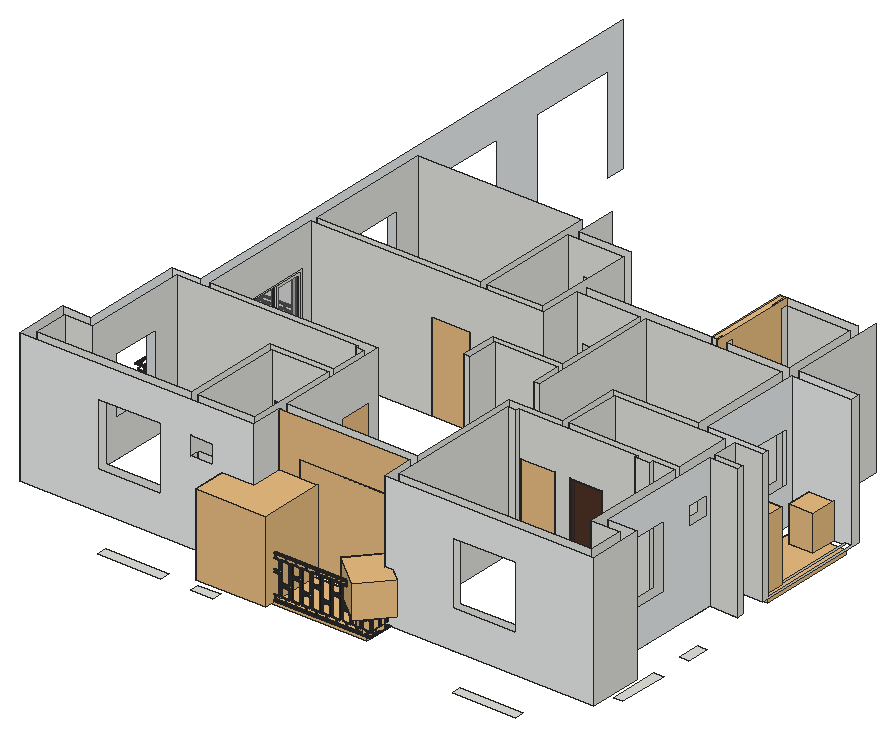
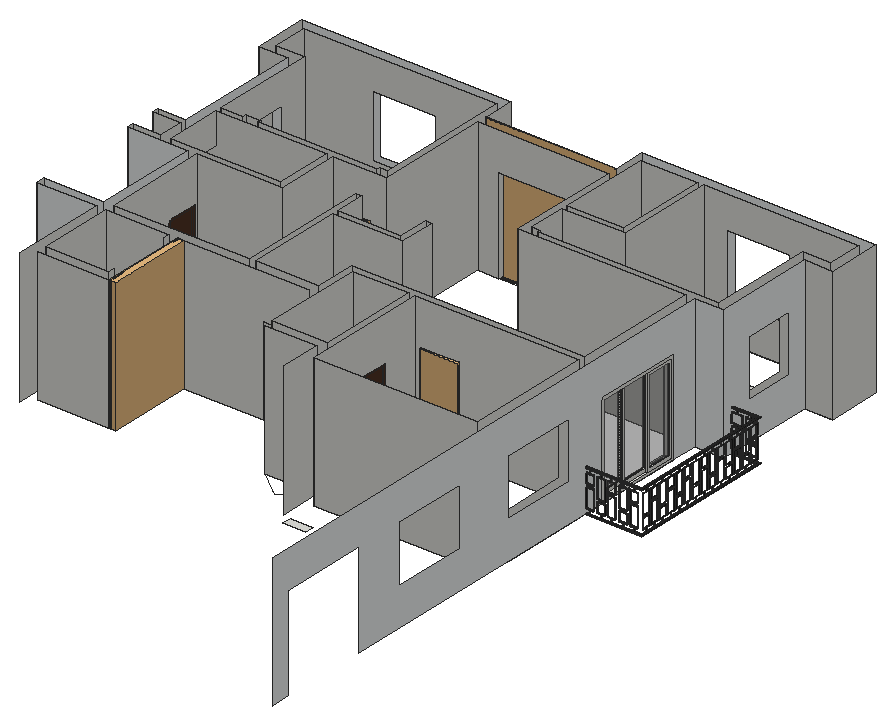
# SketchUp Ruby script. Lengths in inches.
U = 1.inch
M = Sketchup.active_model
def pt(a) = Geom::Point3d.new(a.map { |v| v * U })
def face(e, loops, mat)
  f = e.add_face(loops[0].map { |a| pt(a) })
  loops[1..].each { |l| e.add_face(l.map { |a| pt(a) }).erase! }
  f.material = f.back_material = mat if mat
  f
end
# faces: each face lists its corners as indices into pts; further lists are holes
def faces(e, pts, list, mat = nil) = list.each { |f| face(e, (f[0].is_a?(Array) ? f : [f]).map { |l| l.map { |i| pts[i] } }, mat) }
# xy, xz, yz: faces in a plane at the given z, y or x. An outline is a flat list of corners, or four numbers for a rectangle; further outlines are holes
def ring(l) = l.size == 4 ? [[l[0], l[1]], [l[2], l[1]], [l[2], l[3]], [l[0], l[3]]] : l.each_slice(2).to_a
def flat(e, list, mat, &to3) = list.each { |f| face(e, (f[0].is_a?(Array) ? f : [f]).map { |l| ring(l).map { |u, v| to3.(u, v) } }, mat) }
def xy(e, z, list, mat = nil) = flat(e, list, mat) { |x, y| [x, y, z] }
def xz(e, y, list, mat = nil) = flat(e, list, mat) { |x, z| [x, y, z] }
def yz(e, x, list, mat = nil) = flat(e, list, mat) { |y, z| [x, y, z] }
def lines(e, pts, list) = list.each { |a, b| e.add_line(pt(pts[a]), pt(pts[b])) }
# prism: a flat outline (further loops are holes) pulled along v
def prism(e, loops, v, mat = nil)
  f = face(e, loops, mat); d = Geom::Vector3d.new(v.map { |x| x * U })
  f.pushpull(f.normal.samedirection?(d) ? d.length : -d.length)
end
def box(e, o, s, mat = nil) = prism(e, [[o, [o[0] + s[0], o[1], o[2]], [o[0] + s[0], o[1] + s[1], o[2]], [o[0], o[1] + s[1], o[2]]]], [0, 0, s[2]], mat)
def at(x, y, z, deg = 0) = Geom::Transformation.translation(pt([x, y, z])) * Geom::Transformation.rotation(ORIGIN, Z_AXIS, deg.degrees)
def axes(o, x, y, z) = Geom::Transformation.new([*x, 0, *y, 0, *z, 0, *pt(o).to_a, 1])
def part(name) = M.definitions.add(name)
# library, detail: a bought-in or finely detailed component or shape, given as its bounding box
def library(name, o, s) = part(name).tap { |d| box(d.entities, o, s) }
def detail(e, o, s) = box(e.add_group.entities, o, s)
def put(e, d, t, mat = nil) = e.add_instance(d, t).tap { |i| i.material = mat if mat }
def group(e, t, mat = nil) = e.add_group.tap { |g| g.transformation = t; g.material = mat if mat }.entities
root = M.entities
M.materials.add("02 - Default").color = [196, 209, 187]
M.materials.add("02 - DefaultW").color = [91, 118, 29]
M.materials.add("04 - Default").color = [38, 38, 38]
M.materials.add("04 - DefaultW").color = [92, 55, 26]
M.materials.add("06 - Default").color = [255, 255, 255]
M.materials.add("07 - Default").color = [92, 55, 26]
M.materials.add("10 - Default").color = [62, 56, 39]
M.materials.add("Polis06_194").color = [79, 50, 36]
M.materials.add("[3P0081_White-City]").color = [235, 238, 238]
M.materials.add("[Color M00]").color = [255, 255, 255]
M.materials.add("[Color M08]").color = [30, 30, 30]
M.materials.add("[Translucent Glass Gray]").color = [128, 128, 128]
M.materials["[Translucent Glass Gray]"].alpha = 0.5
c1 = part("Group\#70")
prism(c1.entities,[[[4.13,0,3.9375],[7.875,0,3.9375],[7.875,0,13.78],[4.13,0,13.78],[4.13,0,15.75],[7.875,0,15.75],[7.875,0,35.43],[4.13,0,35.43],[4.13,0,39.37],[3.74,0,39.37],[3.74,0,35.43],[0,0,35.43],[0,0,15.75],[3.74,0,15.75],[3.74,0,13.78],[0,0,13.78],[0,0,3.9375],[3.74,0,3.9375],[3.74,0,0],[4.13,0,0]],[[0.39,0,16.14],[0.39,0,35.04],[7.48,0,35.04],[7.48,0,16.14]],[[7.48,0,4.33],[0.39,0,4.33],[0.39,0,13.39],[7.48,0,13.39]]],[0,0.39,0],"[Color M08]")
c2 = part("Group\#69")
prism(c2.entities,[[[3.74,0,35.43],[0,0,35.43],[0,0,25.59],[3.74,0,25.59],[3.74,0,23.62],[0,0,23.62],[0,0,3.9375],[3.74,0,3.9375],[3.74,0,0],[4.13,0,0],[4.13,0,3.9375],[7.875,0,3.9375],[7.875,0,23.62],[4.13,0,23.62],[4.13,0,25.59],[7.875,0,25.59],[7.875,0,35.43],[4.13,0,35.43],[4.13,0,39.37],[3.74,0,39.37]],[[7.48,0,23.23],[7.48,0,4.33],[0.39,0,4.33],[0.39,0,23.23]],[[0.39,0,35.04],[7.48,0,35.04],[7.48,0,25.98],[0.39,0,25.98]]],[0,0.39,0],"[Color M08]")
c3 = part("Group\#71")
put(c3.entities,c1,at(0,0,0))
put(c3.entities,c2,at(9.84,0,0))
c4 = part("Group\#81")
g1 = group(c4.entities,at(0,0,0))
prism(g1,[[[24,-19.7,0],[0,-19.7,0],[0,120.08,0],[24,120.08,0],[24,118.11,0],[1.97,118.11,0],[1.97,-17.76,0],[24,-17.76,0]]],[0,0,0.79],"[Color M08]")
put(c4.entities,c3,axes([0.79,40.35,0.79],[0,1,0],[1,0,0],[0,0,1]))
put(c4.entities,c3,at(2.95,118.9,0.79))
put(c4.entities,c3,axes([0.79,79.72,0.79],[0,1,0],[1,0,0],[0,0,1]))
put(c4.entities,c3,axes([0.79,60.04,0.79],[0,1,0],[1,0,0],[0,0,1]))
put(c4.entities,c3,axes([0.79,99.41,0.79],[0,1,0],[1,0,0],[0,0,1]))
put(c4.entities,c3,axes([0.79,0.98,0.79],[0,1,0],[1,0,0],[0,0,1]))
g2 = group(c4.entities,at(0,0,40.16))
prism(g2,[[[24,-19.7,0],[0,-19.7,0],[0,120.08,0],[24,120.08,0],[24,118.11,0],[1.97,118.11,0],[1.97,-17.76,0],[24,-17.76,0]]],[0,0,0.79],"[Color M08]")
put(c4.entities,c3,axes([0.79,20.67,0.79],[0,1,0],[1,0,0],[0,0,1]))
put(c4.entities,c3,axes([0.79,-18.7,0.79],[0,1,0],[1,0,0],[0,0,1]))
put(c4.entities,c3,axes([2.95,-18.49,0.79],[1,0,0],[0,-1,0],[0,0,1]))
c5 = library("MONSTERA_Defintion",[-100.72,-132.16,0],[226.75,232.88,1000])
c6 = library("MONSTERA_Defintion1",[-382.23,-503.1,29.34],[811.96,1000,773.77])
c7 = library("POT_Defintion",[-467.71,-467.71,0],[935.42,935.42,1000])
c8 = library("POT_Defintion6",[-504.36,-499.05,1069.94],[1000,1000,51.81])
c9 = library("TABLE_Defintion5",[-349.98,-500,-99.29],[912.18,1000,162.92])
c10 = library("TABLE_Defintion3",[-282.7,-491.23,-690.5],[848.82,1000,669.35])
c11 = library("TABLE_Defintion",[-354.24,-500,-9.27],[914.7,1000,77.28])
c12 = part("Monstera Plant 50")
g3 = group(c12.entities,at(0,0,0))
g4 = group(g3,at(0,0,0))
put(g4,c5,axes([-70.21,316.62,1332.52],[0.60525,0.72131,0],[-0.72131,0.60525,0],[0,0,0.92363]),"02 - DefaultW")
put(g4,c6,axes([-70.21,316.62,1332.52],[2.09136,2.49238,0],[-2.49238,2.09136,0],[0,0,3.1915]),"02 - Default")
g5 = group(c12.entities,at(0,0,0))
g6 = group(g5,at(0,0,0))
put(g6,c7,axes([-63.73,311.08,962.21],[0.47902,0.57088,0],[-0.57088,0.47902,0],[0,0,0.69328]),"04 - Default")
put(g6,c8,axes([-63.73,311.08,962.21],[0.41695,0.4969,0],[-0.4969,0.41695,0],[0,0,0.60345]),"10 - Default")
g7 = group(c12.entities,at(0,0,0))
g8 = group(g7,at(0,0,0))
put(g8,c9,axes([-8.95,303.3125,886.6],[1.07163,-0.6187,0],[0.6187,1.07163,0],[0,0,1.23741]),"04 - DefaultW")
put(g8,c10,axes([-8.95,303.3125,886.6],[1.11435,-0.64337,0],[0.64337,1.11435,0],[0,0,1.28674]),"07 - Default")
put(g8,c11,axes([-8.95,303.3125,886.6],[1.10303,-0.63684,0],[0.63684,1.10303,0],[0,0,1.27367]),"06 - Default")
c13 = library("Flora+17",[-57.52,158.6,-38.64],[66.99,62.88,77.28])
c14 = library("Floor panel",[0,13.98,-0.38],[148.62,177.51,16.92])
c15 = library("Group\#241",[0,-0.25,0],[124.5,0.25,126])
c16 = library("SLIDING+GLASS+DOOR",[0,-0.75,0],[72,5.75,80])
c17 = part("Flush door")
xy(c17.entities,0,[[0,0,4.72,1.18],[0,34.25,4.72,35.43]],"Polis06_194")
xy(c17.entities,85.26,[[0,1.18,4.72,34.25]],"Polis06_194")
xy(c17.entities,86.61,[[0,0,4.72,35.43]],"Polis06_194")
xz(c17.entities,0,[[0,0,4.72,86.61]],"Polis06_194")
xz(c17.entities,1.18,[[0,0,2.36,85.26],[2.36,0,4.72,85.26]],"Polis06_194")
xz(c17.entities,34.25,[[0,0,4.72,85.26]],"Polis06_194")
xz(c17.entities,35.43,[[0,0,4.72,86.61]],"Polis06_194")
yz(c17.entities,0,[[0,0,1.18,86.61],[34.25,0,35.43,86.61],[1.18,85.26,34.25,86.61]],"Polis06_194")
yz(c17.entities,2.36,[[1.18,0,34.25,0,34.25,85.21,1.18,85.26]],"Polis06_194")
yz(c17.entities,4.72,[[0,0,1.18,86.61],[34.25,0,35.43,86.61],[1.18,85.26,34.25,86.61]],"Polis06_194")
c18 = library("PINTU 6 YA",[0,-0.6875,0],[35.83,8.07,80.71])
c19 = part("Group\#75")
put(c19.entities,c1,at(0,0,0))
put(c19.entities,c2,at(9.84,0,0))
c20 = part("Group\#76")
put(c20.entities,c1,at(0,0,0))
put(c20.entities,c2,at(9.84,0,0))
c21 = part("Group\#74")
put(c21.entities,c19,axes([0.79,60.04,0.79],[0,1,0],[1,0,0],[0,0,1]))
put(c21.entities,c19,axes([0.79,40.35,0.79],[0,1,0],[1,0,0],[0,0,1]))
put(c21.entities,c19,axes([0.79,79.72,0.79],[0,1,0],[1,0,0],[0,0,1]))
g9 = group(c21.entities,at(0,0,40.16))
prism(g9,[[[54,-20.92,0],[0,-20.92,0],[0,120.08,0],[27,120.08,0],[27,118.11,0],[1.97,118.11,0],[1.97,-18.98,0],[54,-18.98,0]]],[0,0,0.79],"[Color M08]")
put(c21.entities,c20,axes([0.79,0.98,0.79],[0,1,0],[1,0,0],[0,0,1]))
put(c21.entities,c19,axes([0.79,20.67,0.79],[0,1,0],[1,0,0],[0,0,1]))
put(c21.entities,c19,axes([2.95,118.9,0.79],[1.35733,0,0],[0,1,0],[0,0,1]))
g10 = group(c21.entities,at(0,0,0))
prism(g10,[[[54,-20.92,0],[0,-20.92,0],[0,120.08,0],[27,120.08,0],[27,118.11,0],[1.97,118.11,0],[1.97,-18.98,0],[54,-18.98,0]]],[0,0,0.79],"[Color M08]")
put(c21.entities,c3,axes([0.79,99.41,0.79],[0,1,0],[1,0,0],[0,0,1]))
put(c21.entities,c20,axes([0.79,-18.7,0.79],[0,1,0],[1,0,0],[0,0,1]))
put(c21.entities,c20,axes([22.01,-20.17,0.79],[-1,0,0],[0,1,0],[0,0,1]))
g11 = group(c21.entities,at(43.22,-20.17,0.79))
put(g11,c1,axes([0,0,0],[-1,0,0],[0,1,0],[0,0,1]))
put(g11,c2,axes([-9.84,0,0],[-1,0,0],[0,1,0],[0,0,1]))
put(g11,c2,axes([10.78,0,0],[-1,0,0],[0,1,0],[0,0,1]))
c22 = part("구성 요소\#2")
prism(c22.entities,[[[0,0,0],[118.11,0,0],[118.11,0,78.74],[0,0,78.74]],[[116.14,0,76.77],[116.14,0,1.97],[1.97,0,1.97],[1.97,0,76.77]]],[0,7.875,0])
c23 = part("구성 요소\#1")
xy(c23.entities,0,[[[0,0,40.16,74.8],[2.375,2.375,37.78,72.43]]])
xy(c23.entities,1.18,[[2.375,2.375,37.78,72.43]],"[Translucent Glass Gray]")
xy(c23.entities,2.36,[[[0,0,40.16,74.8],[2.375,2.375,37.78,72.43]]])
xz(c23.entities,0,[[0,0,40.16,2.36]],"[Color M00]")
xz(c23.entities,2.375,[[2.375,0,37.78,1.18],[2.375,1.18,37.78,2.36]])
xz(c23.entities,72.43,[[2.375,0,37.78,1.18],[2.375,1.18,37.78,2.36]])
xz(c23.entities,74.8,[[0,0,40.16,2.36]],"[Color M00]")
yz(c23.entities,0,[[0,0,74.8,2.36]])
yz(c23.entities,2.375,[[2.375,0,72.43,1.18],[2.375,1.18,72.43,2.36]])
yz(c23.entities,37.78,[[2.375,0,72.43,1.18],[2.375,1.18,72.43,2.36]])
yz(c23.entities,40.16,[[0,0,74.8,2.36]])
c24 = part("구성 요소\#3")
xy(c24.entities,0,[[0,0,40.16,2.36]],"[Color M00]")
xy(c24.entities,2.375,[[2.375,0,37.78,1.18],[2.375,1.18,37.78,2.36]])
xy(c24.entities,35.83,[[38.48,0,39.47,0.39]])
xy(c24.entities,35.83,[[38.48,1.97,39.47,2.36]],"[Color M00]")
xy(c24.entities,38.98,[[38.48,0,39.47,0.39]])
xy(c24.entities,38.98,[[38.48,1.97,39.47,2.36]],"[Color M00]")
xy(c24.entities,72.43,[[2.375,0,37.78,1.18],[2.375,1.18,37.78,2.36]])
xy(c24.entities,74.8,[[0,0,40.16,2.36]],"[Color M00]")
xz(c24.entities,0,[[[0,0,40.16,74.8],[2.375,2.375,37.78,72.43],[38.48,35.83,39.47,38.98]]])
xz(c24.entities,0.39,[[38.48,35.83,39.47,38.98]])
xz(c24.entities,1.18,[[2.375,2.375,37.78,72.43]],"[Translucent Glass Gray]")
xz(c24.entities,1.97,[[38.48,35.83,39.47,38.98]],"[Color M00]")
xz(c24.entities,2.36,[[[0,0,40.16,74.8],[2.375,2.375,37.78,72.43],[38.48,35.83,39.47,38.98]]])
yz(c24.entities,0,[[0,0,2.36,74.8]])
yz(c24.entities,2.375,[[0,2.375,1.18,72.43],[1.18,2.375,2.36,72.43]])
yz(c24.entities,37.78,[[0,2.375,1.18,72.43],[1.18,2.375,2.36,72.43]])
yz(c24.entities,38.48,[[0,35.83,0.39,38.98]])
yz(c24.entities,38.48,[[1.97,35.83,2.36,38.98]],"[Color M00]")
yz(c24.entities,39.47,[[0,35.83,0.39,38.98]])
yz(c24.entities,39.47,[[1.97,35.83,2.36,38.98]],"[Color M00]")
yz(c24.entities,40.16,[[0,0,2.36,74.8]])
c25 = part("구성 요소\#4")
put(c25.entities,c23,axes([37.78,4.72,0],[1,0,0],[0,0,1],[0,-1,0]))
put(c25.entities,c24,at(75.5625,0,0))
put(c25.entities,c23,axes([0,7.09,0],[1,0,0],[0,0,1],[0,-1,0]))
c26 = part("그룹\#1")
put(c26.entities,c22,axes([0,0,0],[1.04,0,0],[0,1,0],[0,0,1]))
put(c26.entities,c25,axes([1.97,0.39,1.97],[1.02677,0,0],[0,1,0],[0,0,1]))
c27 = part("sliding door")
put(c27.entities,c26,at(0,0,0))
c28 = library("Scara cu plante",[-7.66,-9.41,-0.15],[30.59,22.83,66.38])
c29 = library("Gruppo\#3",[0,0,0],[23.62,24.19,33.46])
c30 = library("Group\#2",[0,-3.15,0.41],[58,18.09,114.05])
xy(root,228,[[218,357.97,278,366.97],[306,357.97,327.5,366.97],[554.5,357.97,614.5,366.97],[652.5,426.87,661.5,474.87],[652.5,504.97,661.5,526.53],
  [382.75,726.97,404.25,735.97]])
xy(root,264,[[144,357.97,144,408.97,171,408.97,171,428.87,180,428.87,180,399.97,153,399.97,153,366.97,218,366.97,218,357.97],[218,357.97,220,366.97],[220,357.97,276,361.97],[276,357.97,276,366.97,300,366.97,300,459.97,309,459.97,309,453.97,306,453.97,306,357.97],[306,357.97,308,366.97],
  [308,357.97,325.5,361.97],[325.5,357.97,327.5,366.97],[554.5,357.97,556.5,366.97],[556.5,357.97,612.5,361.97],[612.5,357.97,614.5,366.97],
  [614.5,357.97,614.5,366.97,679.5,366.97,679.5,399.97,652.5,399.97,652.5,426.87,661.5,426.87,661.5,408.97,688.5,408.97,688.5,357.97],[220,361.97,276,362.97],[308,361.97,325.5,362.97],[556.5,361.97,612.5,362.97],[220,362.97,276,366.97],
  [308,362.97,325.5,366.97],[556.5,362.97,612.5,366.97],[652.5,426.87,661.5,428.87],[171,428.87,175,472.87],[175,428.87,176,472.87],
  [176,428.87,180,472.87],[652.5,428.87,656.5,472.87],[656.5,428.87,657.5,472.87],[657.5,428.87,661.5,472.87],[171,472.87,180,474.87],
  [652.5,472.87,661.5,474.87],[171,474.87,171,504.97,198,504.97,198,530.97,207,530.97,207,504.97,366,504.97,366,492.97,360,492.97,360,495.97,352,495.97,352,498.97,180,498.97,180,474.87],[539,498.97,539,504.97,541.5,504.97,541.5,564.97,622.5,564.97,622.5,567.97,631.5,567.97,631.5,564.97,688.5,564.97,688.5,558.97,661.5,558.97,661.5,535,688.5,535,688.5,529,661.5,529,661.5,524.53,652.5,524.53,652.5,558.97,547.5,558.97,547.5,504.97,553.5,504.97,553.5,498.97],[652.5,504.97,661.5,505.03],[652.5,505.03,661.5,507.03],
  [652.5,507.03,656.5,524.53],[656.5,507.03,657.5,524.53],[657.5,507.03,661.5,524.53],[198,614.97,198,656.97,207,656.97,207,630.97,321,630.97,321,624.97,207,624.97,207,614.97],[198,656.97,202,724.97],
  [202,656.97,203,724.97],[203,656.97,207,724.97],[553.5,675.97,562.5,741.97],[198,724.97,207,726.97],[384.75,726.97,402.25,730.97],
  [402.25,726.97,404.25,735.97],[384.75,730.97,402.25,731.97],[384.75,731.97,402.25,735.97]])
xz(root,357.97,[[[144,264,366,390],[218,300,278,360],[306,342,327.5,360]],[[490.5,264,688.5,390],[554.5,300,614.5,360]]],"[3P0081_White-City]")
xz(root,366.97,[[[153,264,300,390],[218,300,278,360]],[306,264,306,342,327.5,342,327.5,360,306,360,306,390,360,390,360,264],[[496.5,264,679.5,390],[554.5,300,614.5,360]]])
xz(root,387.97,[[366,264,386.25,264,386.25,354,470.25,354,470.25,264,490.5,264,490.5,390,366,390]],"[3P0081_White-City]")
xz(root,396.97,[[366,264,366,390,490.5,390,490.5,264,470.25,264,470.25,354,386.25,354,386.25,264]])
xz(root,399.97,[[153,264,180,390],[652.5,264,679.5,390]])
xz(root,408.97,[[144,264,171,390],[661.5,264,688.5,390]])
xz(root,453.97,[[306,264,309,264,309,348,333,348,333,264,360,264,360,390,306,390]])
xz(root,459.97,[[300,264,300,390,360,390,360,264,333,264,333,348,309,348,309,264]])
xz(root,462.97,[[360,264,366,348]])
xz(root,492.97,[[360,264,366,348]])
xz(root,495.97,[[352,264,360,390],[496.5,264,504.5,390],[617.5,264,631.5,390]])
xz(root,498.97,[[180,264,352,390],[504.5,264,507,264,507,348,539,348,539,264,553.5,264,553.5,348,583.5,348,583.5,264,617.5,264,617.5,390,504.5,390],[631.5,264,652.5,390]])
xz(root,504.97,[[207,264,366,390],[490.5,264,490.5,390,541.5,390,541.5,264,539,264,539,348,507,348,507,264],[547.5,264,547.5,390,652.5,390,652.5,360,661.5,360,661.5,342,652.5,342,652.5,264,583.5,264,583.5,348,553.5,348,553.5,264]])
xz(root,504.97,[[171,264,198,390]],"[3P0081_White-City]")
xz(root,529,[[661.5,264,688.5,390]])
xz(root,530.97,[[198,264,207,354]])
xz(root,535,[[661.5,264,688.5,390]])
xz(root,537.97,[[421.5,264,427.5,390],[487.5,264,493.5,390]])
xz(root,558.97,[[547.5,264,652.5,390],[661.5,264,688.5,390]])
xz(root,564.97,[[541.5,264,622.5,390]])
xz(root,564.97,[[631.5,264,631.5,390,688.5,390,688.5,266,682.5,266,682.5,264]],"[3P0081_White-City]")
xz(root,566.47,[[427.5,264,487.5,390]])
xz(root,567.97,[[622.5,264,631.5,348]])
xz(root,572.47,[[421.5,264,487.5,390]])
xz(root,597.97,[[622.5,264,631.5,348]])
xz(root,600.97,[[493.5,264,513.5,300]])
xz(root,606.97,[[493.5,264,513.5,300]])
xz(root,614.97,[[198,264,207,354]])
xz(root,624.97,[[207,264,321,264,321,348,357,348,357,264,427.5,264,427.5,390,207,390]])
xz(root,630.97,[[207,264,207,390,363,390,363,264,357,264,357,348,321,348,321,264],[369,264,421.5,390]])
xz(root,663.97,[[427.5,264,433.5,264,433.5,348,472.5,348,472.5,264,487.5,264,487.5,390,427.5,390],[493.5,264,622.5,390]])
xz(root,663.97,[[631.5,264,682.5,264,682.5,266,688.5,266,688.5,390,631.5,390]],"[3P0081_White-City]")
xz(root,666.97,[[363,264,369,348]])
xz(root,672.97,[[430.5,264,430.5,390,553.5,390,553.5,264,472.5,264,472.5,348,433.5,348,433.5,264],[562.5,264,622.5,390]])
xz(root,672.97,[[631.5,264,688.5,390]],"[3P0081_White-City]")
xz(root,690.97,[[363,264,369,348]])
xz(root,726.97,[[[369,264,421.5,390],[382.75,342,404.25,360]]])
xz(root,735.97,[[[372,264,421.5,390],[382.75,342,404.25,360]]])
xz(root,744.97,[[562.5,264,622.5,390]])
xz(root,750.97,[[207,264,363,390]])
xz(root,753.97,[[553.5,264,622.5,390]])
yz(root,144,[[357.97,264,408.97,390]])
yz(root,153,[[366.97,264,399.97,390]])
yz(root,171,[[[408.97,264,504.97,390],[426.87,300,474.87,354]]],"[3P0081_White-City]")
yz(root,180,[[[399.97,264,498.97,390],[426.87,300,474.87,354]]])
yz(root,198,[[[504.97,264,504.97,390,1005.97,390,1005.97,264,987.97,264,987.97,354,903.97,354,903.97,264,614.97,264,614.97,354,530.97,354,530.97,264],[654.97,300,726.97,354],[783.97,300,855.97,354]]],"[3P0081_White-City]")
yz(root,207,[[504.97,264,530.97,264,530.97,354,614.97,354,614.97,264,624.97,264,624.97,390,504.97,390],[[630.97,264,750.97,390],[654.97,300,726.97,354]]])
yz(root,300,[[366.97,264,459.97,390]])
yz(root,306,[[366.97,264,453.97,264,453.97,390,366.97,390,366.97,360,357.97,360,357.97,342,366.97,342]])
yz(root,309,[[453.97,264,459.97,348]])
yz(root,321,[[624.97,264,630.97,348]])
yz(root,333,[[453.97,264,459.97,348]])
yz(root,352,[[495.97,264,498.97,390]])
yz(root,357,[[624.97,264,630.97,348]])
yz(root,360,[[366.97,264,453.97,390],[459.97,264,459.97,390,495.97,390,495.97,264,492.97,264,492.97,348,462.97,348,462.97,264]])
yz(root,363,[[630.97,264,630.97,390,750.97,390,750.97,264,690.97,264,690.97,348,666.97,348,666.97,264]])
yz(root,366,[[357.97,264,387.97,390],[396.97,264,462.97,264,462.97,348,492.97,348,492.97,264,504.97,264,504.97,390,396.97,390]])
yz(root,369,[[630.97,264,666.97,264,666.97,348,690.97,348,690.97,264,726.97,264,726.97,390,630.97,390]])
yz(root,372,[[735.97,264,774.97,390]])
yz(root,386.25,[[387.97,264,396.97,354]])
yz(root,421.5,[[537.97,264,572.47,390],[630.97,264,726.97,390]])
yz(root,427.5,[[537.97,264,566.47,390],[624.97,264,663.97,390]])
yz(root,433.5,[[663.97,264,672.97,348]])
yz(root,470.25,[[387.97,264,396.97,354]])
yz(root,472.5,[[663.97,264,672.97,348]])
yz(root,487.5,[[537.97,264,566.47,390],[572.47,264,663.97,390]])
yz(root,490.5,[[357.97,264,387.97,390],[396.97,264,504.97,390]])
yz(root,493.5,[[537.97,264,600.97,264,600.97,300,606.97,300,606.97,264,663.97,264,663.97,390,537.97,390]])
yz(root,496.5,[[366.97,264,495.97,390]])
yz(root,504.5,[[495.97,264,498.97,390]])
yz(root,507,[[498.97,264,504.97,348]])
yz(root,513.5,[[600.97,264,606.97,300]])
yz(root,539,[[498.97,264,504.97,348]])
yz(root,541.5,[[504.97,264,564.97,390]])
yz(root,547.5,[[504.97,264,558.97,390]])
yz(root,553.5,[[498.97,264,504.97,348],[672.97,264,672.97,390,678.97,390,678.97,266,738.97,266,738.97,390,753.97,390,753.97,264]])
yz(root,562.5,[[672.97,264,741.97,264,741.97,266,678.97,266,678.97,390,672.97,390],[741.97,264,744.97,264,744.97,390,738.97,390,738.97,266,741.97,266]])
yz(root,583.5,[[498.97,264,504.97,348]])
yz(root,617.5,[[495.97,264,498.97,390]])
yz(root,622.5,[[[564.97,264,564.97,390,663.97,390,663.97,264,597.97,264,597.97,348,567.97,348,567.97,264],[609.97,300,657.97,348]],[672.97,264,744.97,390]])
yz(root,631.5,[[495.97,264,498.97,390],[672.97,264,763.97,390]])
yz(root,631.5,[[[564.97,264,567.97,264,567.97,348,597.97,348,597.97,264,663.97,264,663.97,390,564.97,390],[609.97,300,657.97,348]]],"[3P0081_White-City]")
yz(root,652.5,[[[399.97,264,498.97,390],[426.87,300,474.87,360]],[504.97,264,504.97,342,526.53,342,526.53,360,504.97,360,504.97,390,558.97,390,558.97,264]])
yz(root,661.5,[[535,264,558.97,390]])
yz(root,661.5,[[[408.97,264,529,390],[426.87,300,474.87,360],[504.97,342,526.53,360]]],"[3P0081_White-City]")
yz(root,679.5,[[366.97,264,399.97,390]])
yz(root,682.5,[[564.97,264,663.97,266]])
yz(root,688.5,[[357.97,264,408.97,390],[529,264,535,390],[558.97,264,672.97,264,672.97,390,663.97,390,663.97,266,564.97,266,564.97,390,558.97,390]])
p = [[144,635.47,264],[198,635.47,264],[201.5,587.47,264],[201.5,585.97,264],[198,530.97,264],[198,532.97,264],
  [200.5,612.97,264],[200.5,585.97,264],[207,614.97,264],[207,612.97,264],[201.5,558.97,264],[202.5,558.97,264],
  [198,612.97,264],[202.5,587.47,264],[207,532.97,264],[203.5,532.97,264],[406.25,391.97,264],[446.25,391.97,264],
  [470.25,387.97,264],[468.25,387.97,264],[388.25,387.97,264],[388.25,396.97,264],[446.25,392.97,264],[203.5,559.97,264],
  [427.25,392.97,264],[421.5,624.97,264],[421.5,572.47,264],[598.5,597.97,264],[598.5,639.97,264],[202.5,559.97,264],
  [406.25,392.97,264],[468.25,393.97,264],[427.25,393.97,264],[622.5,597.97,264],[468.25,396.97,264],[386.25,396.97,264],
  [541.5,558.97,264],[493.5,558.97,264],[541.5,564.97,264],[493.5,564.97,264],[306,498.97,264],[306,459.97,264],
  [341,692.97,264],[363,692.97,264],[341,750.97,264],[487.5,537.97,264],[487.5,504.97,264],[511.5,606.97,264],
  [511.5,639.97,264],[300,498.97,264],[300,459.97,264],[427.5,624.97,264],[427.5,572.47,264],[493.5,537.97,264],
  [493.5,504.97,264],[396.75,755.47,264],[421.5,735.97,264],[372,735.97,264],[202.5,532.97,264],[468.25,392.97,264],
  [207,530.97,264],[201.5,612.97,264],[386.25,387.97,264],[487.5,546.47,264],[427.5,546.47,264],[198,614.97,264],
  [175,366.97,264],[175,399.97,264],[470.25,396.97,264],[657.5,366.97,264],[657.5,399.97,264],[474.5,572.47,264],
  [474.5,663.97,264]]
lines(root,p,[[0,1],[2,3],[4,5],[6,7],[8,9],[10,11],[12,6],[7,3],[13,2],[14,15],[16,17],[18,19],
  [20,21],[17,22],[15,23],[24,22],[25,26],[27,28],[29,11],[30,16],[31,32],[27,33],[23,29],[34,31],
  [35,21],[32,24],[36,37],[38,39],[40,41],[42,43],[44,42],[45,46],[47,48],[28,48],[49,50],[51,52],
  [53,54],[55,56],[55,57],[11,58],[9,14],[3,10],[24,30],[59,19],[14,60],[29,13],[61,9],[5,12],
  [6,61],[15,58],[58,5],[2,61],[21,34],[22,59],[19,20],[31,59],[20,62],[63,64],[12,65],[66,67],
  [34,68],[69,70],[71,72]])
put(root,c4,axes([477.26,333.97,264],[0,1,0],[-0.97654,0,0],[0,0,1]))
put(root,c12,axes([483.73,342.98,263.46],[0.01275,0,0],[0,0.01275,0],[0,0,0.01275]))
put(root,c13,at(393.59,167.58,300))
put(root,c14,axes([496.83,339.97,256.54],[0,0.30278,0],[-0.66754,0,0],[0,0,0.27]))
put(root,c15,at(366,387.97,264))
put(root,c16,axes([386.25,387.97,264],[1.16667,0,0],[0,1,0],[0,0,1.125]))
put(root,c17,axes([333,458.7,264],[0,-1,0],[-0.67733,0,0],[0,0,0.96982]))
put(root,c18,axes([365.3125,462.99,264],[0.01802,0.8369,0],[-0.99977,0.02153,0],[0,0,1.04078]))
put(root,c17,axes([583.5,504.39,264],[0,-1,0],[-0.84667,0,0],[0,0,0.96982]))
put(root,c18,axes([539,499.66,264],[-0.89311,0,0],[0,1,0],[0,0,1.04078]))
put(root,c21,axes([144,614.55,264],[1,0,0],[0,-1,0],[0,0,0.97692]))
put(root,c27,axes([198,614.97,264],[0,-0.68385,0],[1,0,0],[0,0,1.143]))
put(root,c28,axes([660.01,578.41,264],[1,0,0],[0,-1,0],[0,0,1]))
put(root,c17,axes([627.22,597.97,264],[-1,0,0],[0,-0.84667,0],[0,0,0.96982]))
put(root,c14,axes([637.5,560.65,258.32],[0.32297,0,0],[0,0.52389,0],[0,0,0.27]))
put(root,c18,axes([321,625.66,264],[1.00475,0,0],[0,1,0],[0,0,1.04078]))
put(root,c29,at(647.91,639.78,264))
put(root,c17,axes([367.72,690.97,264],[-1,0,0],[0,-0.67733,0],[0,0,0.96982]))
put(root,c30,axes([549.76,753.97,263.54],[0,-1.39655,0],[0.34,0,0],[0,0,1.10484]))
